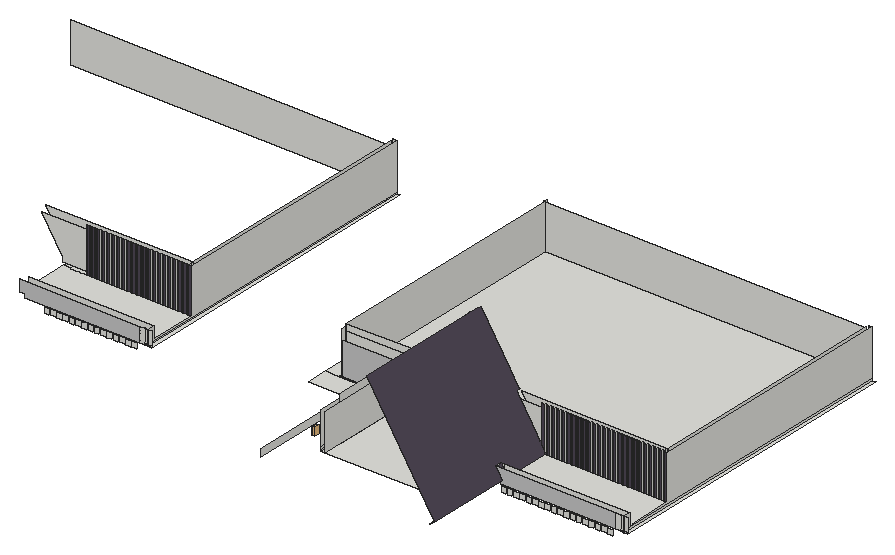
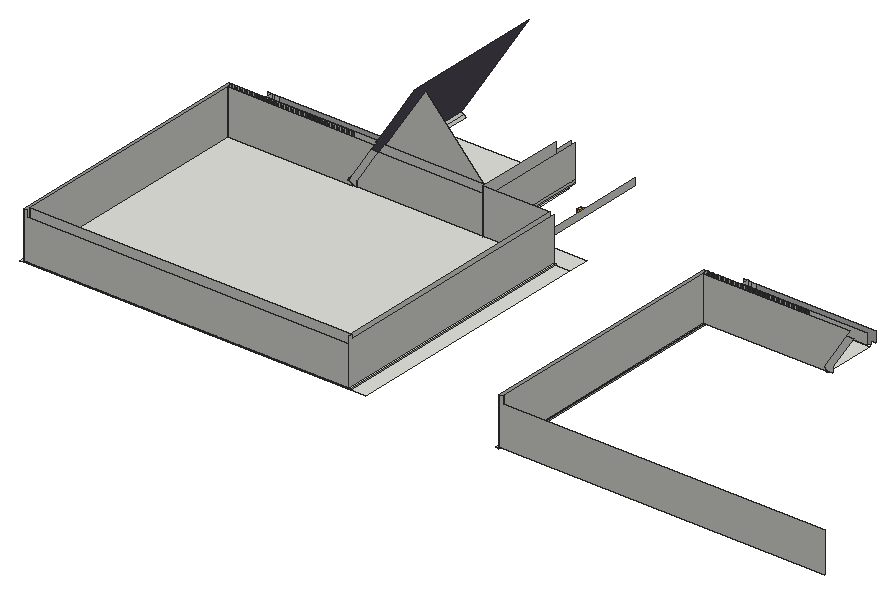
# SketchUp Ruby script. Lengths in inches.
U = 1.inch
M = Sketchup.active_model
def pt(a) = Geom::Point3d.new(a.map { |v| v * U })
def face(e, loops, mat)
  f = e.add_face(loops[0].map { |a| pt(a) })
  loops[1..].each { |l| e.add_face(l.map { |a| pt(a) }).erase! }
  f.material = f.back_material = mat if mat
  f
end
# faces: each face lists its corners as indices into pts; further lists are holes
def faces(e, pts, list, mat = nil) = list.each { |f| face(e, (f[0].is_a?(Array) ? f : [f]).map { |l| l.map { |i| pts[i] } }, mat) }
# xy, xz, yz: faces in a plane at the given z, y or x. An outline is a flat list of corners, or four numbers for a rectangle; further outlines are holes
def ring(l) = l.size == 4 ? [[l[0], l[1]], [l[2], l[1]], [l[2], l[3]], [l[0], l[3]]] : l.each_slice(2).to_a
def flat(e, list, mat, &to3) = list.each { |f| face(e, (f[0].is_a?(Array) ? f : [f]).map { |l| ring(l).map { |u, v| to3.(u, v) } }, mat) }
def xy(e, z, list, mat = nil) = flat(e, list, mat) { |x, y| [x, y, z] }
def xz(e, y, list, mat = nil) = flat(e, list, mat) { |x, z| [x, y, z] }
def yz(e, x, list, mat = nil) = flat(e, list, mat) { |y, z| [x, y, z] }
def lines(e, pts, list) = list.each { |a, b| e.add_line(pt(pts[a]), pt(pts[b])) }
# prism: a flat outline (further loops are holes) pulled along v
def prism(e, loops, v, mat = nil)
  f = face(e, loops, mat); d = Geom::Vector3d.new(v.map { |x| x * U })
  f.pushpull(f.normal.samedirection?(d) ? d.length : -d.length)
end
def box(e, o, s, mat = nil) = prism(e, [[o, [o[0] + s[0], o[1], o[2]], [o[0] + s[0], o[1] + s[1], o[2]], [o[0], o[1] + s[1], o[2]]]], [0, 0, s[2]], mat)
def at(x, y, z, deg = 0) = Geom::Transformation.translation(pt([x, y, z])) * Geom::Transformation.rotation(ORIGIN, Z_AXIS, deg.degrees)
def axes(o, x, y, z) = Geom::Transformation.new([*x, 0, *y, 0, *z, 0, *pt(o).to_a, 1])
def part(name) = M.definitions.add(name)
# library, detail: a bought-in or finely detailed component or shape, given as its bounding box
def library(name, o, s) = part(name).tap { |d| box(d.entities, o, s) }
def detail(e, o, s) = box(e.add_group.entities, o, s)
def put(e, d, t, mat = nil) = e.add_instance(d, t).tap { |i| i.material = mat if mat }
def group(e, t, mat = nil) = e.add_group.tap { |g| g.transformation = t; g.material = mat if mat }.entities
root = M.entities
M.materials.add("[Color M02]").color = [198, 198, 198]
M.materials.add("[Color M06]").color = [79, 71, 84]
M.materials.add("[Color M07]").color = [58, 58, 58]
c1 = library("Group\#13",[0,0,0],[3.54,3.54,3.9375])
xy(root,240.47,[[2236.57,591.8125,2240.94,646.3125],[2240.94,591.8125,2251.71,646.3125]])
xy(root,251.0625,[[2251.71,562.32,2251.71,732.32,2085.33,732.32,2085.33,1195.68,2683.5,1195.68,2683.5,630.04,2444.26,630.04,2444.26,562.32],[2208.71,567.01,2219.52,646.3125],[2219.52,567.01,2236.57,646.3125],[2236.57,567.01,2236.57,646.3125,2219.52,646.3125,2219.52,732.32,2251.71,732.32,2251.71,567.01],[1803.23,623.84,1810.23,1201.875],
  [2683.5,623.84,2683.5,1195.68,2085.33,1195.68,2085.33,732.32,2208.71,732.32,2208.71,726.125,2197.32,726.125,2197.32,686.3125,2135.95,686.3125,2135.95,726.125,2079.13,726.125,2079.13,1201.875,2689.7,1201.875,2689.7,623.84],[2689.7,623.84,2696.7,1201.875],[2197.32,646.3125,2208.71,726.125],[2208.71,646.3125,2219.52,732.32],[2051.88,686.3125,2135.95,726.125],
  [2051.88,726.125,2079.13,1201.875]])
xy(root,253.4375,[[2202.51,541.0625,2208.71,541.0625,2208.71,732.32,2085.33,732.32,2085.33,1195.68,2683.5,1195.68,2683.5,623.84,2689.7,623.84,2689.7,1201.875,2082.95,1201.875,2082.95,726.125,2135.95,726.125,2135.95,686.3125,2202.51,686.3125],[2079.13,726.125,2082.95,1201.875]])
xy(root,257.0625,[[2444.39,521.5625,2450.46,726.125],[2200.93,528.48,2208.71,719.59],[2208.71,528.48,2209.43,719.59],[2209.43,528.48,2444.39,719.59],[1563.99,636.82,1803.23,636.82,1803.23,724.8125,1797.15,724.8125,1797.15,726.125,1793.73,726.125,1793.73,724.8125,1787.65,724.8125,1787.65,726.125,1784.23,726.125,1784.23,724.8125,1778.15,724.8125,1778.15,726.125,1774.73,726.125,1774.73,724.8125,1768.65,724.8125,1768.65,726.125,1765.23,726.125,1765.23,724.8125,1759.15,724.8125,1759.15,726.125,1755.73,726.125,1755.73,724.8125,1749.65,724.8125,1749.65,726.125,1746.23,726.125,1746.23,724.8125,1740.15,724.8125,1740.15,726.125,1736.73,726.125,1736.73,724.8125,1730.65,724.8125,1730.65,726.125,1727.23,726.125,1727.23,724.8125,1721.15,724.8125,1721.15,726.125,1717.73,726.125,1717.73,724.8125,1711.65,724.8125,1711.65,726.125,1708.23,726.125,1708.23,724.8125,1702.15,724.8125,1702.15,726.125,1698.73,726.125,1698.73,724.8125,1692.65,724.8125,1692.65,726.125,1689.23,726.125,1689.23,724.8125,1683.15,724.8125,1683.15,726.125,1679.73,726.125,1679.73,724.8125,1673.65,724.8125,1673.65,726.125,1670.23,726.125,1670.23,724.8125,1664.15,724.8125,1664.15,726.125,1660.73,726.125,1660.73,724.8125,1654.65,724.8125,1654.65,726.125,1651.23,726.125,1651.23,724.8125,1645.15,724.8125,1645.15,726.125,1641.73,726.125,1641.73,724.8125,1635.65,724.8125,1635.65,726.125,1632.23,726.125,1632.23,724.8125,1626.15,724.8125,1626.15,726.125,1622.73,726.125,1622.73,724.8125,1616.65,724.8125,1616.65,726.125,1613.23,726.125,1613.23,724.8125,1607.15,724.8125,1607.15,726.125,1603.73,726.125,1603.73,724.8125,1597.65,724.8125,1597.65,726.125,1594.23,726.125,1594.23,724.8125,1588.15,724.8125,1588.15,726.125,1584.73,726.125,1584.73,724.8125,1578.65,724.8125,1578.65,726.125,1563.99,726.125],
  [2450.46,636.82,2689.7,636.82,2689.7,724.8125,2683.62,724.8125,2683.62,726.125,2680.2,726.125,2680.2,724.8125,2674.12,724.8125,2674.12,726.125,2670.7,726.125,2670.7,724.8125,2664.62,724.8125,2664.62,726.125,2661.2,726.125,2661.2,724.8125,2655.12,724.8125,2655.12,726.125,2651.7,726.125,2651.7,724.8125,2645.62,724.8125,2645.62,726.125,2642.2,726.125,2642.2,724.8125,2636.12,724.8125,2636.12,726.125,2632.7,726.125,2632.7,724.8125,2626.62,724.8125,2626.62,726.125,2623.2,726.125,2623.2,724.8125,2617.12,724.8125,2617.12,726.125,2613.7,726.125,2613.7,724.8125,2607.62,724.8125,2607.62,726.125,2604.2,726.125,2604.2,724.8125,2598.12,724.8125,2598.12,726.125,2594.7,726.125,2594.7,724.8125,2588.62,724.8125,2588.62,726.125,2585.2,726.125,2585.2,724.8125,2579.12,724.8125,2579.12,726.125,2575.7,726.125,2575.7,724.8125,2569.62,724.8125,2569.62,726.125,2566.2,726.125,2566.2,724.8125,2560.12,724.8125,2560.12,726.125,2556.7,726.125,2556.7,724.8125,2550.62,724.8125,2550.62,726.125,2547.2,726.125,2547.2,724.8125,2541.12,724.8125,2541.12,726.125,2537.7,726.125,2537.7,724.8125,2531.62,724.8125,2531.62,726.125,2528.2,726.125,2528.2,724.8125,2522.12,724.8125,2522.12,726.125,2518.7,726.125,2518.7,724.8125,2512.62,724.8125,2512.62,726.125,2509.2,726.125,2509.2,724.8125,2503.12,724.8125,2503.12,726.125,2499.7,726.125,2499.7,724.8125,2493.62,724.8125,2493.62,726.125,2490.2,726.125,2490.2,724.8125,2484.12,724.8125,2484.12,726.125,2480.7,726.125,2480.7,724.8125,2474.62,724.8125,2474.62,726.125,2471.2,726.125,2471.2,724.8125,2465.12,724.8125,2465.12,726.125,2450.46,726.125],[2202.51,719.59,2208.71,726.125],[2208.71,719.59,2209.43,726.125],[2209.43,719.59,2444.39,726.125],[1578.65,724.8125,1578.65,726.125,1563.99,726.125,1563.99,732.2,1797.15,732.2,1797.15,726.125,1793.73,726.125,1793.73,724.8125,1787.65,724.8125,1787.65,726.125,1784.23,726.125,1784.23,724.8125,1778.15,724.8125,1778.15,726.125,1774.73,726.125,1774.73,724.8125,1768.65,724.8125,1768.65,726.125,1765.23,726.125,1765.23,724.8125,1759.15,724.8125,1759.15,726.125,1755.73,726.125,1755.73,724.8125,1749.65,724.8125,1749.65,726.125,1746.23,726.125,1746.23,724.8125,1740.15,724.8125,1740.15,726.125,1736.73,726.125,1736.73,724.8125,1730.65,724.8125,1730.65,726.125,1727.23,726.125,1727.23,724.8125,1721.15,724.8125,1721.15,726.125,1717.73,726.125,1717.73,724.8125,1711.65,724.8125,1711.65,726.125,1708.23,726.125,1708.23,724.8125,1702.15,724.8125,1702.15,726.125,1698.73,726.125,1698.73,724.8125,1692.65,724.8125,1692.65,726.125,1689.23,726.125,1689.23,724.8125,1683.15,724.8125,1683.15,726.125,1679.73,726.125,1679.73,724.8125,1673.65,724.8125,1673.65,726.125,1670.23,726.125,1670.23,724.8125,1664.15,724.8125,1664.15,726.125,1660.73,726.125,1660.73,724.8125,1654.65,724.8125,1654.65,726.125,1651.23,726.125,1651.23,724.8125,1645.15,724.8125,1645.15,726.125,1641.73,726.125,1641.73,724.8125,1635.65,724.8125,1635.65,726.125,1632.23,726.125,1632.23,724.8125,1626.15,724.8125,1626.15,726.125,1622.73,726.125,1622.73,724.8125,1616.65,724.8125,1616.65,726.125,1613.23,726.125,1613.23,724.8125,1607.15,724.8125,1607.15,726.125,1603.73,726.125,1603.73,724.8125,1597.65,724.8125,1597.65,726.125,1594.23,726.125,1594.23,724.8125,1588.15,724.8125,1588.15,726.125,1584.73,726.125,1584.73,724.8125],
  [2465.12,724.8125,2465.12,726.125,2450.46,726.125,2450.46,732.2,2683.62,732.2,2683.62,726.125,2680.2,726.125,2680.2,724.8125,2674.12,724.8125,2674.12,726.125,2670.7,726.125,2670.7,724.8125,2664.62,724.8125,2664.62,726.125,2661.2,726.125,2661.2,724.8125,2655.12,724.8125,2655.12,726.125,2651.7,726.125,2651.7,724.8125,2645.62,724.8125,2645.62,726.125,2642.2,726.125,2642.2,724.8125,2636.12,724.8125,2636.12,726.125,2632.7,726.125,2632.7,724.8125,2626.62,724.8125,2626.62,726.125,2623.2,726.125,2623.2,724.8125,2617.12,724.8125,2617.12,726.125,2613.7,726.125,2613.7,724.8125,2607.62,724.8125,2607.62,726.125,2604.2,726.125,2604.2,724.8125,2598.12,724.8125,2598.12,726.125,2594.7,726.125,2594.7,724.8125,2588.62,724.8125,2588.62,726.125,2585.2,726.125,2585.2,724.8125,2579.12,724.8125,2579.12,726.125,2575.7,726.125,2575.7,724.8125,2569.62,724.8125,2569.62,726.125,2566.2,726.125,2566.2,724.8125,2560.12,724.8125,2560.12,726.125,2556.7,726.125,2556.7,724.8125,2550.62,724.8125,2550.62,726.125,2547.2,726.125,2547.2,724.8125,2541.12,724.8125,2541.12,726.125,2537.7,726.125,2537.7,724.8125,2531.62,724.8125,2531.62,726.125,2528.2,726.125,2528.2,724.8125,2522.12,724.8125,2522.12,726.125,2518.7,726.125,2518.7,724.8125,2512.62,724.8125,2512.62,726.125,2509.2,726.125,2509.2,724.8125,2503.12,724.8125,2503.12,726.125,2499.7,726.125,2499.7,724.8125,2493.62,724.8125,2493.62,726.125,2490.2,726.125,2490.2,724.8125,2484.12,724.8125,2484.12,726.125,2480.7,726.125,2480.7,724.8125,2474.62,724.8125,2474.62,726.125,2471.2,726.125,2471.2,724.8125],[2209.43,726.125,2444.39,732.2],[2444.39,726.125,2450.46,732.2],[1563.99,732.2,1797.15,734.4375],[2085.21,732.2,2450.46,732.2,2450.46,734.4375,2683.62,734.4375,2683.62,1195.8,2085.21,1195.8],
  [2450.46,732.2,2683.62,734.4375]])
xz(root,620.37,[[1612.66,240.88,1621.34,251.0625],[1624.34,240.88,1633.03,251.0625],[1636.03,240.88,1644.72,251.0625],[1647.72,240.88,1656.41,251.0625],[1659.41,240.88,1668.09,251.0625],
  [1671.09,240.88,1679.78,251.0625],[1682.78,240.88,1691.47,251.0625],[1694.47,240.88,1703.16,251.0625],[1706.16,240.88,1714.84,251.0625],[1717.84,240.88,1726.53,251.0625],
  [1729.53,240.88,1738.22,251.0625],[1741.22,240.88,1749.91,251.0625],[1752.91,240.88,1761.59,251.0625],[1764.59,240.88,1773.28,251.0625],[1776.28,240.88,1784.97,251.0625],
  [2464.06,240.88,2472.75,251.0625],[2475.75,240.88,2484.43,251.0625],[2487.43,240.88,2496.12,251.0625],[2499.12,240.88,2507.81,251.0625],[2510.81,240.88,2519.5,251.0625],
  [2522.5,240.88,2531.18,251.0625],[2534.18,240.88,2542.87,251.0625],[2545.87,240.88,2554.56,251.0625],[2557.56,240.88,2566.25,251.0625],[2569.25,240.88,2577.93,251.0625],
  [2580.93,240.88,2589.62,251.0625],[2592.62,240.88,2601.31,251.0625],[2604.31,240.88,2613,251.0625],[2616,240.88,2624.68,251.0625],[2627.68,240.88,2636.37,251.0625],
  [2639.37,240.88,2648.06,251.0625],[2651.06,240.88,2659.75,251.0625],[2662.75,240.88,2671.43,251.0625]])
xz(root,623.84,[[1787.6875,251.0625,1797.03,278.1875],[1797.03,251.0625,1803.23,253.4375],[1803.23,251.0625,1810.23,253.4375],[2674.15,251.0625,2683.5,278.1875],[2683.5,251.0625,2689.7,253.4375],
  [2689.7,251.0625,2696.7,253.4375],[1797.03,253.4375,1803.23,278.1875],[1803.23,253.4375,1810.23,278.1875],[2683.5,253.4375,2689.7,278.1875],[2689.7,253.4375,2696.7,278.1875]])
xz(root,623.84,[[1573.31,251.0625,1787.6875,251.0625,1787.6875,278.1875,1563.99,278.1875,1563.99,257.0625,1573.31,257.0625],[2459.77,251.0625,2674.15,251.0625,2674.15,278.1875,2450.46,278.1875,2450.46,257.0625,2459.77,257.0625]],"[Color M02]")
xz(root,636.82,[[1569.71,257.0625,1803.23,278.1875],[2450.46,257.0625,2456.17,278.1875],[2456.17,257.0625,2689.7,278.1875]])
xz(root,686.3125,[[2135.95,251.0625,2202.51,253.4375]])
xz(root,719.59,[[2200.93,257.0625,2202.51,258.95],[2202.51,257.0625,2202.51,263.89,2200.93,263.89,2200.93,326.08,2209.43,326.08,2209.43,257.0625],[2209.43,257.0625,2444.39,257.0625,2444.39,266.53,2326.48,450.4375,2232.12,350.1875,2222.65,340.125,2209.43,326.08],[2200.93,258.95,2202.51,263.89]])
xz(root,724.8125,[[1607.15,257.0625,1613.23,340.125],[1616.65,257.0625,1622.73,340.125],[1626.15,257.0625,1632.23,340.125],[1635.65,257.0625,1641.73,340.125],[1645.15,257.0625,1651.23,340.125],
  [1654.65,257.0625,1660.73,340.125],[1664.15,257.0625,1670.23,340.125],[1673.65,257.0625,1679.73,340.125],[1683.15,257.0625,1689.23,340.125],[1692.65,257.0625,1698.73,340.125],
  [1702.15,257.0625,1708.23,340.125],[1711.65,257.0625,1717.73,340.125],[1721.15,257.0625,1727.23,340.125],[1730.65,257.0625,1736.73,340.125],[1740.15,257.0625,1746.23,340.125],
  [1749.65,257.0625,1755.73,340.125],[1759.15,257.0625,1765.23,340.125],[1768.65,257.0625,1774.73,340.125],[1778.15,257.0625,1784.23,340.125],[1787.65,257.0625,1793.73,340.125],
  [1797.15,257.0625,1803.23,340.125],[2465.12,257.0625,2471.2,340.125],[2474.62,257.0625,2480.7,340.125],[2484.12,257.0625,2490.2,340.125],[2493.62,257.0625,2499.7,340.125],
  [2503.12,257.0625,2509.2,340.125],[2512.62,257.0625,2518.7,340.125],[2522.12,257.0625,2528.2,340.125],[2531.62,257.0625,2537.7,340.125],[2541.12,257.0625,2547.2,340.125],
  [2550.62,257.0625,2556.7,340.125],[2560.12,257.0625,2566.2,340.125],[2569.62,257.0625,2575.7,340.125],[2579.12,257.0625,2585.2,340.125],[2588.62,257.0625,2594.7,340.125],
  [2598.12,257.0625,2604.2,340.125],[2607.62,257.0625,2613.7,340.125],[2617.12,257.0625,2623.2,340.125],[2626.62,257.0625,2632.7,340.125],[2636.12,257.0625,2642.2,340.125],
  [2645.62,257.0625,2651.7,340.125],[2655.12,257.0625,2661.2,340.125],[2664.62,257.0625,2670.7,340.125],[2674.12,257.0625,2680.2,340.125],[2683.62,257.0625,2689.7,340.125],
  [2461.7,260.03,2461.7,340.125,2455.62,340.125,2455.62,269.51,2455.72,269.35,2459.77,263.03]],"[Color M06]")
xz(root,726.125,[[2079.13,251.0625,2135.95,253.4375],[2197.32,251.0625,2208.71,251.0625,2208.71,257.0625,2202.51,257.0625,2202.51,258.95,2197.32,258.95],[2453.7,252.01,2450.46,257.0625,2456.17,257.0625,2457.75,254.61],[2457.75,254.61,2456.17,257.0625,2461.57,257.0625],[2209.43,257.0625,2436.62,257.0625,2436.62,278.65,2397.21,340.125,2209.43,340.125],
  [2436.62,257.0625,2442.7,257.0625,2442.7,269.17,2436.62,278.65],[2442.7,257.0625,2446.12,257.0625,2446.12,263.83,2444.39,266.53,2442.7,269.17],[2446.12,257.0625,2450.46,257.0625,2446.12,263.83],[2450.46,257.0625,2450.46,265.98,2446.12,272.75,2446.12,263.83],[2450.46,257.0625,2452.2,257.0625,2452.2,258.18],
  [2450.46,257.0625,2452.2,258.18,2452.2,263.27,2450.46,265.98],[2452.2,257.0625,2455.62,257.0625,2455.62,257.93,2454.51,259.66,2452.2,258.18],[2455.62,257.0625,2456.17,257.0625,2455.62,257.93],[2456.17,257.0625,2461.57,257.0625,2461.7,257.14,2461.7,260.03,2459.77,263.03,2455.62,260.37,2455.62,257.93],[2461.57,257.0625,2461.7,257.0625,2461.7,257.14],
  [2461.7,257.14,2463.01,257.98,2461.7,260.03],[2455.62,257.93,2455.62,260.37,2454.51,259.66],[2452.2,258.18,2454.51,259.66,2452.2,263.27],[2135.95,258.95,2197.32,263.89],[2197.32,258.95,2202.51,263.89],
  [2454.51,259.66,2455.62,260.37,2455.62,269.29,2452.2,267.09,2452.2,263.27],[2455.62,260.37,2459.77,263.03,2455.72,269.35,2455.62,269.29],[2452.2,263.27,2452.2,267.09,2450.46,265.98],[2446.12,263.83,2446.12,272.75,2442.7,278.09,2442.7,269.17,2444.39,266.53],[2197.32,263.89,2202.51,315.25]])
xz(root,726.125,[[2082.95,253.4375,2135.95,253.4375,2135.95,263.89,2197.32,263.89,2197.32,315.25,2082.95,315.25]],"[Color M02]")
xz(root,726.125,[[1613.23,257.0625,1616.65,340.125],[1622.73,257.0625,1626.15,340.125],[1632.23,257.0625,1635.65,340.125],[1641.73,257.0625,1645.15,340.125],[1651.23,257.0625,1654.65,340.125],
  [1660.73,257.0625,1664.15,340.125],[1670.23,257.0625,1673.65,340.125],[1679.73,257.0625,1683.15,340.125],[1689.23,257.0625,1692.65,340.125],[1698.73,257.0625,1702.15,340.125],
  [1708.23,257.0625,1711.65,340.125],[1717.73,257.0625,1721.15,340.125],[1727.23,257.0625,1730.65,340.125],[1736.73,257.0625,1740.15,340.125],[1746.23,257.0625,1749.65,340.125],
  [1755.73,257.0625,1759.15,340.125],[1765.23,257.0625,1768.65,340.125],[1774.73,257.0625,1778.15,340.125],[1784.23,257.0625,1787.65,340.125],[1793.73,257.0625,1797.15,340.125],
  [2461.7,257.0625,2465.12,257.0625,2465.12,340.125,2461.7,340.125,2461.7,260.03,2463.01,257.98,2461.7,257.14],[2471.2,257.0625,2474.62,340.125],[2480.7,257.0625,2484.12,340.125],[2490.2,257.0625,2493.62,340.125],[2499.7,257.0625,2503.12,340.125],
  [2509.2,257.0625,2512.62,340.125],[2518.7,257.0625,2522.12,340.125],[2528.2,257.0625,2531.62,340.125],[2537.7,257.0625,2541.12,340.125],[2547.2,257.0625,2550.62,340.125],
  [2556.7,257.0625,2560.12,340.125],[2566.2,257.0625,2569.62,340.125],[2575.7,257.0625,2579.12,340.125],[2585.2,257.0625,2588.62,340.125],[2594.7,257.0625,2598.12,340.125],
  [2604.2,257.0625,2607.62,340.125],[2613.7,257.0625,2617.12,340.125],[2623.2,257.0625,2626.62,340.125],[2632.7,257.0625,2636.12,340.125],[2642.2,257.0625,2645.62,340.125],
  [2651.7,257.0625,2655.12,340.125],[2661.2,257.0625,2664.62,340.125],[2670.7,257.0625,2674.12,340.125],[2680.2,257.0625,2683.62,340.125]],"[Color M06]")
xz(root,732.2,[[1557.92,257.0625,1557.92,266.53,1518.52,328,1797.03,328,1797.03,340.125,1797.15,340.125,1797.15,257.0625],[2085.21,257.0625,2209.43,328],[2209.43,257.0625,2209.43,326.08,2211.23,328,2404.98,328,2444.39,266.53,2444.39,257.0625],[2444.39,257.0625,2444.39,266.53,2404.98,328,2683.5,328,2683.5,340.125,2683.62,340.125,2683.62,257.0625]])
xz(root,732.32,[[2085.33,251.0625,2208.71,253.4375],[2085.33,253.4375,2208.71,340.125]])
xz(root,734.4375,[[1563.99,257.0625,1568.05,259.66,1573.31,263.03,1569.26,269.35,1563.99,277.56,1523.88,340.125,1797.15,340.125,1797.15,257.0625],[2450.46,257.0625,2454.51,259.66,2459.77,263.03,2455.72,269.35,2450.46,277.56,2410.35,340.125,2683.62,340.125,2683.62,257.0625]])
xz(root,1195.68,[[2085.33,251.0625,2683.5,253.4375],[2085.33,253.4375,2683.5,340.125]])
xz(root,1201.875,[[2079.13,251.0625,2689.7,253.4375],[1196.48,253.4375,1196.48,328,1797.03,328,1797.03,340.125,1803.23,340.125,1803.23,253.4375],[2082.95,253.4375,2082.95,328,2683.5,328,2683.5,340.125,2689.7,340.125,2689.7,253.4375]])
yz(root,1607.15,[[724.8125,257.0625,726.125,340.125]])
yz(root,1613.23,[[724.8125,257.0625,726.125,340.125]])
yz(root,1616.65,[[724.8125,257.0625,726.125,340.125]])
yz(root,1622.73,[[724.8125,257.0625,726.125,340.125]])
yz(root,1626.15,[[724.8125,257.0625,726.125,340.125]])
yz(root,1632.23,[[724.8125,257.0625,726.125,340.125]])
yz(root,1635.65,[[724.8125,257.0625,726.125,340.125]])
yz(root,1641.73,[[724.8125,257.0625,726.125,340.125]])
yz(root,1645.15,[[724.8125,257.0625,726.125,340.125]])
yz(root,1651.23,[[724.8125,257.0625,726.125,340.125]])
yz(root,1654.65,[[724.8125,257.0625,726.125,340.125]])
yz(root,1660.73,[[724.8125,257.0625,726.125,340.125]])
yz(root,1664.15,[[724.8125,257.0625,726.125,340.125]])
yz(root,1670.23,[[724.8125,257.0625,726.125,340.125]])
yz(root,1673.65,[[724.8125,257.0625,726.125,340.125]])
yz(root,1679.73,[[724.8125,257.0625,726.125,340.125]])
yz(root,1683.15,[[724.8125,257.0625,726.125,340.125]])
yz(root,1689.23,[[724.8125,257.0625,726.125,340.125]])
yz(root,1692.65,[[724.8125,257.0625,726.125,340.125]])
yz(root,1698.73,[[724.8125,257.0625,726.125,340.125]])
yz(root,1702.15,[[724.8125,257.0625,726.125,340.125]])
yz(root,1708.23,[[724.8125,257.0625,726.125,340.125]])
yz(root,1711.65,[[724.8125,257.0625,726.125,340.125]])
yz(root,1717.73,[[724.8125,257.0625,726.125,340.125]])
yz(root,1721.15,[[724.8125,257.0625,726.125,340.125]])
yz(root,1727.23,[[724.8125,257.0625,726.125,340.125]])
yz(root,1730.65,[[724.8125,257.0625,726.125,340.125]])
yz(root,1736.73,[[724.8125,257.0625,726.125,340.125]])
yz(root,1740.15,[[724.8125,257.0625,726.125,340.125]])
yz(root,1746.23,[[724.8125,257.0625,726.125,340.125]])
yz(root,1749.65,[[724.8125,257.0625,726.125,340.125]])
yz(root,1755.73,[[724.8125,257.0625,726.125,340.125]])
yz(root,1759.15,[[724.8125,257.0625,726.125,340.125]])
yz(root,1765.23,[[724.8125,257.0625,726.125,340.125]])
yz(root,1768.65,[[724.8125,257.0625,726.125,340.125]])
yz(root,1774.73,[[724.8125,257.0625,726.125,340.125]])
yz(root,1778.15,[[724.8125,257.0625,726.125,340.125]])
yz(root,1784.23,[[724.8125,257.0625,726.125,340.125]])
yz(root,1787.65,[[724.8125,257.0625,726.125,340.125]])
yz(root,1793.73,[[724.8125,257.0625,726.125,340.125]])
yz(root,1797.03,[[623.84,251.0625,630.04,253.4375],[630.04,251.0625,1195.68,253.4375]])
yz(root,1797.15,[[724.8125,257.0625,726.125,340.125],[726.125,257.0625,732.2,340.125],[732.2,257.0625,734.4375,340.125],[734.4375,257.0625,1195.8,340.125]])
yz(root,1803.23,[[623.84,251.0625,1201.875,253.4375],[623.84,253.4375,1201.875,253.4375,1201.875,340.125,724.8125,340.125,724.8125,257.0625,636.82,257.0625,636.82,278.1875,623.84,278.1875]])
yz(root,2079.13,[[726.125,251.0625,1201.875,253.4375]])
yz(root,2082.95,[[726.125,253.4375,726.125,333.125,1195.68,333.125,1195.68,340.125,1201.875,340.125,1201.875,253.4375]])
yz(root,2085.33,[[732.32,251.0625,1195.68,253.4375],[732.32,253.4375,1195.68,340.125]])
yz(root,2135.95,[[469.875,251.0625,469.875,263.89,726.125,263.89,726.125,253.4375,686.3125,253.4375,686.3125,251.0625],[686.3125,251.0625,726.125,253.4375]])
yz(root,2200.93,[[528.48,257.0625,719.59,258.95],[528.48,258.95,719.59,263.89],[528.48,263.89,719.59,326.08]])
yz(root,2202.51,[[719.59,257.0625,726.125,258.95],[719.59,258.95,726.125,263.89]])
yz(root,2208.71,[[562.32,251.0625,726.125,253.4375],[726.125,251.0625,732.32,253.4375],[562.32,253.4375,726.125,257.0625],[726.125,253.4375,732.32,253.4375,732.32,340.125,562.32,340.125,562.32,257.0625,726.125,257.0625]])
yz(root,2209.43,[[528.48,257.0625,719.59,326.08],[719.59,257.0625,726.125,326.08],[726.125,257.0625,732.2,326.08]])
yz(root,2236.57,[[591.8125,240.47,646.3125,251.0625]],"[Color M07]")
yz(root,2444.39,[[528.48,257.0625,719.59,266.53],[719.59,257.0625,732.2,266.53]])
yz(root,2450.46,[[623.84,257.0625,636.82,278.1875]])
yz(root,2461.7,[[724.8125,260.03,726.125,340.125]])
yz(root,2465.12,[[724.8125,257.0625,726.125,340.125]])
yz(root,2471.2,[[724.8125,257.0625,726.125,340.125]])
yz(root,2474.62,[[724.8125,257.0625,726.125,340.125]])
yz(root,2480.7,[[724.8125,257.0625,726.125,340.125]])
yz(root,2484.12,[[724.8125,257.0625,726.125,340.125]])
yz(root,2490.2,[[724.8125,257.0625,726.125,340.125]])
yz(root,2493.62,[[724.8125,257.0625,726.125,340.125]])
yz(root,2499.7,[[724.8125,257.0625,726.125,340.125]])
yz(root,2503.12,[[724.8125,257.0625,726.125,340.125]])
yz(root,2509.2,[[724.8125,257.0625,726.125,340.125]])
yz(root,2512.62,[[724.8125,257.0625,726.125,340.125]])
yz(root,2518.7,[[724.8125,257.0625,726.125,340.125]])
yz(root,2522.12,[[724.8125,257.0625,726.125,340.125]])
yz(root,2528.2,[[724.8125,257.0625,726.125,340.125]])
yz(root,2531.62,[[724.8125,257.0625,726.125,340.125]])
yz(root,2537.7,[[724.8125,257.0625,726.125,340.125]])
yz(root,2541.12,[[724.8125,257.0625,726.125,340.125]])
yz(root,2547.2,[[724.8125,257.0625,726.125,340.125]])
yz(root,2550.62,[[724.8125,257.0625,726.125,340.125]])
yz(root,2556.7,[[724.8125,257.0625,726.125,340.125]])
yz(root,2560.12,[[724.8125,257.0625,726.125,340.125]])
yz(root,2566.2,[[724.8125,257.0625,726.125,340.125]])
yz(root,2569.62,[[724.8125,257.0625,726.125,340.125]])
yz(root,2575.7,[[724.8125,257.0625,726.125,340.125]])
yz(root,2579.12,[[724.8125,257.0625,726.125,340.125]])
yz(root,2585.2,[[724.8125,257.0625,726.125,340.125]])
yz(root,2588.62,[[724.8125,257.0625,726.125,340.125]])
yz(root,2594.7,[[724.8125,257.0625,726.125,340.125]])
yz(root,2598.12,[[724.8125,257.0625,726.125,340.125]])
yz(root,2604.2,[[724.8125,257.0625,726.125,340.125]])
yz(root,2607.62,[[724.8125,257.0625,726.125,340.125]])
yz(root,2613.7,[[724.8125,257.0625,726.125,340.125]])
yz(root,2617.12,[[724.8125,257.0625,726.125,340.125]])
yz(root,2623.2,[[724.8125,257.0625,726.125,340.125]])
yz(root,2626.62,[[724.8125,257.0625,726.125,340.125]])
yz(root,2632.7,[[724.8125,257.0625,726.125,340.125]])
yz(root,2636.12,[[724.8125,257.0625,726.125,340.125]])
yz(root,2642.2,[[724.8125,257.0625,726.125,340.125]])
yz(root,2645.62,[[724.8125,257.0625,726.125,340.125]])
yz(root,2651.7,[[724.8125,257.0625,726.125,340.125]])
yz(root,2655.12,[[724.8125,257.0625,726.125,340.125]])
yz(root,2661.2,[[724.8125,257.0625,726.125,340.125]])
yz(root,2664.62,[[724.8125,257.0625,726.125,340.125]])
yz(root,2670.7,[[724.8125,257.0625,726.125,340.125]])
yz(root,2674.12,[[724.8125,257.0625,726.125,340.125]])
yz(root,2680.2,[[724.8125,257.0625,726.125,340.125]])
yz(root,2683.5,[[623.84,251.0625,630.04,253.4375],[630.04,251.0625,1195.68,253.4375]])
yz(root,2683.62,[[724.8125,257.0625,726.125,340.125],[726.125,257.0625,732.2,340.125],[732.2,257.0625,734.4375,340.125],[734.4375,257.0625,1195.8,340.125]])
yz(root,2689.7,[[623.84,251.0625,1201.875,253.4375],[623.84,253.4375,1201.875,253.4375,1201.875,340.125,724.8125,340.125,724.8125,257.0625,636.82,257.0625,636.82,278.1875,623.84,278.1875]])
p = [[2453.7,719.59,252.01],[2453.7,726.125,252.01],[2457.75,726.125,254.61],[2457.75,467.1875,254.61],[2453.7,467.1875,252.01],[2453.7,521.5625,252.01],
  [2453.7,528.48,252.01],[2453.7,623.84,252.01],[2453.7,636.82,252.01],[2450.46,623.84,257.0625],[2450.46,636.82,257.0625],[2450.46,719.59,257.0625],
  [2450.46,726.125,257.0625],[2461.57,726.125,257.0625],[2461.7,726.125,257.14],[2463.01,726.125,257.98],[2463.01,467.1875,257.98],[2444.39,528.48,266.53],
  [2444.39,719.59,266.53],[2450.46,528.48,257.0625],[2444.39,726.125,266.53],[2446.12,726.125,263.83],[2452.2,726.125,258.18],[2454.51,726.125,259.66],
  [2454.51,734.4375,259.66],[2450.46,734.4375,257.0625],[2450.46,732.2,257.0625],[2335.8,726.125,456.41],[2335.8,467.1875,456.41],[2459.22,467.1875,263.89],
  [2459.77,467.1875,263.03],[2461.7,726.125,260.03],[2461.7,724.8125,260.03],[2459.77,724.8125,263.03],[2455.72,724.8125,269.35],[2455.62,724.8125,269.51],
  [2455.62,726.125,269.51],[2452.2,726.125,274.85],[2452.2,724.8125,274.85],[2450.46,724.8125,277.56],[2446.12,724.8125,284.33],[2446.12,726.125,284.33],
  [2442.7,726.125,289.67],[2442.7,724.8125,289.67],[2436.62,724.8125,299.15],[2436.62,726.125,299.15],[2410.35,726.125,340.125],[2408.18,726.125,343.5],
  [2408.18,732.2,343.5],[2403.9,732.2,350.1875],[2392.28,732.2,368.3125],[2390.61,732.2,370.91],[2335.8,732.2,456.41],[2455.62,726.125,260.37],
  [2459.77,726.125,263.03],[2459.77,734.4375,263.03],[2455.72,726.125,269.35],[2455.72,734.4375,269.35],[2218.7,646.3125,240.47],[2218.7,686.3125,240.47],
  [2450.17,636.82,257.0625]]
faces(root,p,[[0,1,2,3,4,5,6,7,8],[9,10,8,7],[10,11,0,8],[11,12,1,0],[3,2,13,14,15,16],[17,18,11,10,9,19],[11,18,20,21,12],[12,22,23,24,25,26],
  [23,53,54,55,24],[31,54,33,32],[54,56,34,33],[54,56,57,55]])
faces(root,p,[[27,28,29,30,16,15,31,32,33,34,35,36,37,38,39,40,41,42,43,44,45,46,47,48,49,50,51,52]],"[Color M06]")
lines(root,p,[[58,59],[10,60]])
put(root,c1,axes([2151.5,577,258.17],[-1.5535,0,0],[0,2.39,0],[0,0,-3.63878]))
